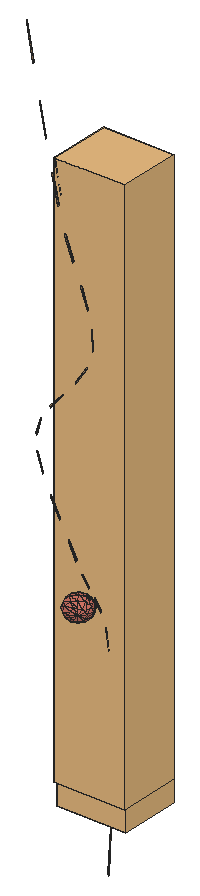
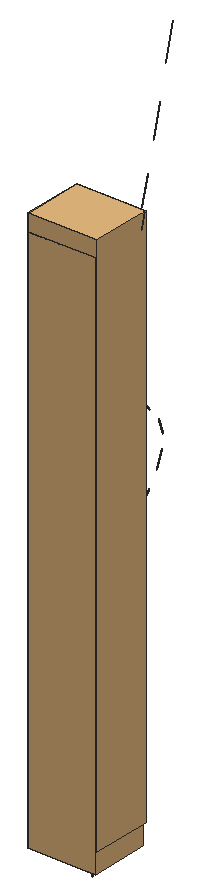
# SketchUp Ruby script. Lengths in inches.
U = 1.inch
M = Sketchup.active_model
def pt(a) = Geom::Point3d.new(a.map { |v| v * U })
def face(e, loops, mat)
  f = e.add_face(loops[0].map { |a| pt(a) })
  loops[1..].each { |l| e.add_face(l.map { |a| pt(a) }).erase! }
  f.material = f.back_material = mat if mat
  f
end
# faces: each face lists its corners as indices into pts; further lists are holes
def faces(e, pts, list, mat = nil) = list.each { |f| face(e, (f[0].is_a?(Array) ? f : [f]).map { |l| l.map { |i| pts[i] } }, mat) }
# xy, xz, yz: faces in a plane at the given z, y or x. An outline is a flat list of corners, or four numbers for a rectangle; further outlines are holes
def ring(l) = l.size == 4 ? [[l[0], l[1]], [l[2], l[1]], [l[2], l[3]], [l[0], l[3]]] : l.each_slice(2).to_a
def flat(e, list, mat, &to3) = list.each { |f| face(e, (f[0].is_a?(Array) ? f : [f]).map { |l| ring(l).map { |u, v| to3.(u, v) } }, mat) }
def xy(e, z, list, mat = nil) = flat(e, list, mat) { |x, y| [x, y, z] }
def xz(e, y, list, mat = nil) = flat(e, list, mat) { |x, z| [x, y, z] }
def yz(e, x, list, mat = nil) = flat(e, list, mat) { |y, z| [x, y, z] }
def lines(e, pts, list) = list.each { |a, b| e.add_line(pt(pts[a]), pt(pts[b])) }
# prism: a flat outline (further loops are holes) pulled along v
def prism(e, loops, v, mat = nil)
  f = face(e, loops, mat); d = Geom::Vector3d.new(v.map { |x| x * U })
  f.pushpull(f.normal.samedirection?(d) ? d.length : -d.length)
end
def box(e, o, s, mat = nil) = prism(e, [[o, [o[0] + s[0], o[1], o[2]], [o[0] + s[0], o[1] + s[1], o[2]], [o[0], o[1] + s[1], o[2]]]], [0, 0, s[2]], mat)
def at(x, y, z, deg = 0) = Geom::Transformation.translation(pt([x, y, z])) * Geom::Transformation.rotation(ORIGIN, Z_AXIS, deg.degrees)
def axes(o, x, y, z) = Geom::Transformation.new([*x, 0, *y, 0, *z, 0, *pt(o).to_a, 1])
def part(name) = M.definitions.add(name)
# library, detail: a bought-in or finely detailed component or shape, given as its bounding box
def library(name, o, s) = part(name).tap { |d| box(d.entities, o, s) }
def detail(e, o, s) = box(e.add_group.entities, o, s)
def put(e, d, t, mat = nil) = e.add_instance(d, t).tap { |i| i.material = mat if mat }
def group(e, t, mat = nil) = e.add_group.tap { |g| g.transformation = t; g.material = mat if mat }.entities
root = M.entities
M.materials.add("green").color = [174, 139, 102]
M.materials.add("vio").color = [206, 114, 100]
c1 = part("3DGeom~157_Defintion")
p = [[36.26,422.52,-32.42],[38.24,377.08,-31.875],[36.84,377.08,-32.625],[36.48,335.72,-32.39],[36.5,298.41,-30.99],[35.18,298.44,-31.7],
  [37.84,335.71,-31.66],[37.69,422.54,-31.65],[32.26,525.68,-30.66],[36.2,472.09,-30.97],[34.73,472.06,-31.76],[33.77,525.72,-29.85],
  [38.91,422.55,-30.49],[40.28,377.08,-29.35],[39.43,377.08,-30.75],[32.92,265.24,-30.5625],[30.44,237.94,-28.41],[29.19,238.08,-29.09],
  [34.2,265.18,-29.87],[39,335.7,-30.56],[38.43,298.38,-28.59],[37.62,298.39,-29.92],[39,335.7,-30.56],[39.83,335.69,-29.19],
  [38.91,422.55,-30.49],[39.79,422.55,-29.05],[35.05,525.75,-28.63],[38.35,472.11,-28.31],[37.45,472.11,-29.79],[35.3,265.14,-28.83],
  [32.28,237.79,-26.11],[31.51,237.83,-27.38],[35.3,265.14,-28.83],[36.08,265.13,-27.54],[35.05,525.75,-28.63],[35.97,525.76,-27.12],
  [23.82,217.46,-27.21],[18.65,200.68,-24.19],[17.48,200.96,-24.87],[25.03,217.22,-26.53],[26.07,217.0625,-25.51],[20.4,200.41,-21.9375],
  [19.66,200.49,-23.18],[26.07,217.0625,-25.51],[26.82,216.99,-24.25],[10.9,186.23,-22.05],[5.93,170.61,-18.08],[4.76,170.8,-18.73],
  [12.06,185.96,-21.38],[13.07,185.79,-20.39],[7.7,170.5,-15.93],[6.95,170.51,-17.12],[13.07,185.79,-20.39],[13.8,185.74,-19.17],
  [20.05,-83.49,-19.57],[20.36,-107.02,-19.07],[19.4,-106.97,-19.5],[21.05,-83.47,-19.125],[21.92,-83.48,-18.41],[21.84,-107.05,-17.47],
  [21.21,-107.04,-18.37],[21.92,-83.48,-18.41],[22.57,-83.5,-17.49],[15.89,-132.25,-16.89],[11.4,-159.71,-12.15],[10.49,-159.62,-12.57],
  [16.82,-132.33,-16.46],[17.65,-132.37,-15.78],[12.79,-159.74,-10.65],[12.19,-159.75,-11.49],[17.65,-132.37,-15.78],[18.26,-132.36,-14.91],
  [8.68,-47.13,-7.48],[17.3,-62.98,-14.9375],[16.31,-63.1,-15.41],[9.65,-46.9375,-6.96],[-0.37,152.09,-14.84],[-4.1,128.9,-8.55],
  [-5.27,128.96,-9.15],[0.82,152,-14.22],[10.53,-46.89,-6.21],[18.84,-63.04,-13.28],[18.18,-62.96,-14.21],[10.53,-46.89,-6.21],
  [11.23,-47.01,-5.28],[1.84,151.98,-13.29],[-2.34,129.04,-6.52],[-3.09,128.93,-7.65],[1.84,151.98,-13.29],[2.59,152.03,-12.12],
  [4.13,-189.34,-7.37],[-1.4,-221.72,-1.7],[-2.26,-221.65,-2.09],[5.01,-189.42,-6.97],[5.79,-189.46,-6.32],[-0.09,-221.74,-0.28],
  [-0.65,-221.75,-1.08],[5.79,-189.46,-6.32],[6.37,-189.45,-5.5],[-10.47,103.92,-1.64],[-14.15,78.09,6.94],[-15.28,78.11,6.38],
  [-9.3125,103.88,-1.06],[-8.3125,103.93,-0.18],[-12.43,78.3,8.88],[-13.16,78.16,7.8],[-8.3125,103.93,-0.18],[-7.57,104.07,0.93],
  [-9.84,-21.39,10.9375],[0.27,-33.63,2.53],[-0.69,-33.86,1.98],[-7.77,-256.8,2.46],[-11.81,-294.96,6.87],[-12.6,-294.92,6.51],
  [-6.94,-256.85,2.84],[-8.85,-21.17,11.49],[-7.96,-21.11,12.28],[1.87,-33.69,4.24],[1.16,-33.57,3.31],[-6.21,-256.87,3.44],
  [-10.59,-294.97,8.17],[-11.11,-294.98,7.4375],[-6.21,-256.87,3.44],[-5.66,-256.86,4.21],[-7.96,-21.11,12.28],[-7.25,-21.21,13.24],
  [-17.49,-335.72,10.65],[-21.71,-379.24,15.19],[-22.42,-379.2,14.875],[-16.73,-335.76,10.98],[-16.07,-335.78,11.53],[-20.62,-379.24,16.37],
  [-21.08,-379.25,15.71],[-16.07,-335.78,11.53],[-15.58,-335.77,12.22],[-19.05,52.72,13.59],[-20.01,29.02,19.21],[-21.11,28.99,18.68],
  [-17.94,52.72,14.13],[-16.97,52.79,14.98],[-18.37,29.18,21.08],[-19.0625,29.08,20.03],[-16.97,52.79,14.98],[-16.26,52.93,16.03],
  [-20.8125,8.25,20.38],[-15.98,-7.82,18.1],[-17.02,-7.99,17.57],[-19.74,8.3125,20.9],[-18.81,8.36,21.71],[-14.38,-7.82,19.9],
  [-15.07,-7.76,18.9],[-27.41,-425.36,19.19],[-31.82,-474.23,23.89],[-32.45,-474.2,23.61],[-26.74,-425.39,19.5],[-18.81,8.36,21.71],
  [-18.13,8.38,22.74],[-26.15,-425.41,19.98],[-30.85,-474.24,24.93],[-31.27,-474.24,24.35],[-26.15,-425.41,19.98],[-25.71,-425.4,20.6]]
faces(c1.entities,p,[[0,1,2],[3,4,5],[3,6,4],[0,7,1],[8,9,10],[8,11,9],[12,13,14],[15,16,17],
  [15,18,16],[19,20,21],[22,23,20],[24,25,13],[26,27,28],[29,30,31],[32,33,30],[34,35,27],
  [36,37,38],[36,39,37],[40,41,42],[43,44,41],[45,46,47],[45,48,46],[49,50,51],[52,53,50],
  [54,55,56],[54,57,55],[58,59,60],[61,62,59],[63,64,65],[63,66,64],[67,68,69],[70,71,68],
  [72,73,74],[72,75,73],[76,77,78],[76,79,77],[80,81,82],[83,84,81],[85,86,87],[88,89,86],
  [90,91,92],[90,93,91],[94,95,96],[97,98,95],[99,100,101],[99,102,100],[103,104,105],[106,107,104],
  [108,109,110],[111,112,113],[111,114,112],[108,115,109],[116,117,118],[119,120,121],[122,123,120],[124,125,117],
  [126,127,128],[126,129,127],[130,131,132],[133,134,131],[135,136,137],[135,138,136],[139,140,141],[142,143,140],
  [144,145,146],[144,147,145],[148,149,150],[151,152,153],[151,154,152],[155,156,149],[157,158,159],[160,161,158]],"green")
c2 = part("3DGeom~246_Defintion")
p = [[52.16,0,-500],[255.625,-213.37,-352.41],[17.91,-184.79,-452.79],[295.17,0,-406.93],[-204.83,0,-459.09],[-224.6,106.69,-431.83],
  [17.91,184.79,-452.79],[-224.6,-106.6875,-431.83],[-406.93,0,-295.17],[-406.93,0,-295.17],[147.59,-369.57,-203.47],[-75.65,-320.06,-323.79],
  [147.59,-369.57,-203.47],[-75.65,-320.06,-323.79],[255.625,213.37,-352.41],[-278.62,184.79,-357.36],[-75.65,320.06,-323.79],[-75.65,-320.06,-323.79],
  [-278.62,-184.79,-357.36],[-278.62,-184.79,-357.36],[-406.93,0,-295.17],[-406.93,0,-295.17],[295.17,0,-406.93],[424.85,-184.79,-157.61],
  [255.625,-213.37,-352.41],[295.17,0,-406.93],[459.09,0,-204.83],[255.625,213.37,-352.41],[295.17,0,-406.93],[-278.62,-184.79,-357.36],
  [-203.47,-369.57,-147.59],[-352.41,-213.37,-255.625],[-278.62,-184.79,-357.36],[-75.65,-320.06,-323.79],[-278.62,-184.79,-357.36],[-352.41,-213.37,-255.625],
  [-406.93,0,-295.17],[-352.41,213.37,-255.625],[-278.62,184.79,-357.36],[-352.41,213.37,-255.625],[-75.65,320.06,-323.79],[-278.62,184.79,-357.36],
  [255.625,-213.37,-352.41],[331.28,-320.06,-28.62],[147.59,-369.57,-203.47],[255.625,-213.37,-352.41],[331.28,-320.06,-28.62],[255.625,213.37,-352.41],
  [424.85,184.79,-157.61],[147.59,369.57,-203.47],[255.625,213.37,-352.41],[147.59,369.57,-203.47],[0,-426.74,0],[147.59,-369.57,-203.47],
  [-352.41,213.37,-255.625],[-203.47,369.57,-147.59],[-75.65,320.06,-323.79],[147.59,369.57,-203.47],[-75.65,320.06,-323.79],[-426.21,-184.79,-153.89],
  [-480.23,-106.6875,-79.42],[-500,0,-52.16],[-480.23,106.6875,-79.42],[-426.21,184.78,-153.89],[-203.47,-369.57,-147.59],[-331.28,-320.06,28.62],
  [-203.47,369.57,-147.59],[480.23,-106.69,79.42],[500,0,52.16],[203.47,-369.57,147.59],[331.28,-320.06,-28.62],[147.59,369.57,-203.47],
  [331.28,320.06,-28.62],[0,426.74,0],[331.28,320.06,-28.62],[147.59,369.57,-203.47],[147.59,369.57,-203.47],[426.21,-184.78,153.89],
  [331.28,-320.06,-28.62],[480.23,106.6875,79.42],[-424.85,-184.78,157.61],[-331.28,320.06,28.62],[-203.47,369.57,-147.59],[-147.59,-369.57,203.47],
  [-147.59,-369.57,203.47],[-331.28,-320.06,28.62],[-331.28,320.06,28.62],[-459.09,0,204.83],[-424.85,184.79,157.61],[331.28,-320.06,-28.62],
  [352.41,-213.37,255.625],[203.47,-369.57,147.59],[331.28,-320.06,-28.62],[426.21,184.79,153.89],[203.47,369.57,147.59],[203.47,369.57,147.59],
  [331.28,320.06,-28.62],[75.65,-320.06,323.79],[-147.59,-369.57,203.47],[75.65,-320.06,323.79],[-331.28,320.06,28.62],[-147.59,369.57,203.47],
  [-147.59,-369.57,203.47],[-255.625,-213.37,352.41],[-147.59,369.57,203.47],[406.93,0,295.17],[278.62,-184.79,357.36],[75.65,-320.06,323.79],
  [352.41,-213.37,255.625],[278.62,-184.79,357.36],[203.47,369.57,147.59],[352.41,213.37,255.625],[75.65,320.06,323.79],[352.41,213.37,255.625],
  [-295.17,0,406.93],[-255.625,213.37,352.41],[-147.59,369.57,203.47],[-147.59,-369.57,203.47],[-17.91,-184.79,452.79],[-255.625,-213.37,352.41],
  [-147.59,-369.57,203.47],[75.65,-320.06,323.79],[-255.625,213.37,352.41],[75.65,320.06,323.79],[-147.59,369.57,203.47],[278.62,-184.79,357.36],
  [278.62,184.79,357.36],[278.62,184.79,357.36],[352.41,213.37,255.625],[224.6,-106.69,431.83],[278.62,-184.79,357.36],[406.93,0,295.17],
  [204.83,0,459.09],[406.93,0,295.17],[224.6,106.6875,431.83],[406.93,0,295.17],[278.62,184.79,357.36],[406.93,0,295.17],
  [-255.625,213.37,352.41],[-17.91,184.79,452.79],[75.65,320.06,323.79],[278.62,184.79,357.36],[75.65,320.06,323.79],[-255.625,-213.37,352.41],
  [-52.16,0,500],[-295.17,0,406.93],[-255.625,-213.37,352.41],[-295.17,0,406.93],[-255.625,213.37,352.41],[278.62,184.79,357.36],
  [-295.17,0,406.93]]
faces(c2.entities,p,[[0,1,2],[0,3,1],[4,0,2],[5,6,0],[5,0,4],[6,3,0],[4,2,7],[4,7,8],
  [5,4,9],[2,10,11],[2,1,12],[7,2,13],[6,14,3],[15,6,5],[15,16,6],[16,14,6],
  [7,17,18],[7,19,20],[15,5,21],[22,23,24],[25,26,23],[27,26,28],[29,30,31],[32,33,30],
  [34,35,36],[37,38,36],[39,40,41],[42,43,44],[45,23,46],[47,48,26],[49,48,50],[16,51,14],
  [33,52,30],[33,53,52],[54,55,56],[55,57,58],[35,59,36],[59,60,36],[60,61,36],[61,62,36],
  [62,63,36],[63,37,36],[35,64,65],[35,65,59],[63,66,37],[26,67,23],[26,68,67],[48,68,26],
  [53,69,52],[53,70,69],[71,72,48],[73,74,75],[55,73,76],[23,77,78],[23,67,77],[48,79,68],
  [72,79,48],[59,65,80],[59,80,60],[62,81,63],[63,81,82],[30,52,83],[30,84,85],[86,73,55],
  [60,80,87],[60,87,61],[61,88,62],[62,88,81],[61,87,88],[89,90,91],[92,77,90],[72,93,79],
  [94,93,72],[73,95,96],[52,97,98],[52,69,99],[100,101,73],[101,95,73],[65,102,103],[65,103,80],
  [88,104,81],[67,68,105],[68,79,105],[77,67,105],[79,93,105],[69,106,107],[69,108,109],[110,111,93],
  [112,113,95],[101,112,95],[90,77,105],[93,111,105],[80,103,114],[80,114,87],[87,115,88],[88,115,116],
  [117,118,119],[120,121,118],[122,123,124],[87,114,115],[125,90,105],[111,126,105],[112,127,128],[129,130,131],
  [132,129,133],[134,132,135],[136,134,137],[121,129,118],[121,130,129],[138,139,140],[139,141,142],[143,144,145],
  [146,118,144],[147,139,148],[139,134,149],[150,144,139],[118,129,132],[144,132,134],[144,134,139],[118,132,144]],"vio")
c3 = part("3DGeom~39_Defintion")
p = [[35.12,-55.5,-54.41],[34.11,-55.53,-54.86],[35.81,-76.47,-55.34],[36.8,-76.41,-54.9],[38.88,-99.33,-54.67],[37.91,-99.4,-55.11],
  [39.32,-123.69,-53.625],[40.28,-123.64,-53.2],[37.08,-24.79,-53.05],[36.07,-24.5,-53.5],[33.89,-37.16,-54.23],[34.93,-37.21,-53.77],
  [44.64,-14.39,-49.98],[39.94,-17.85,-52.2],[40.77,-18.46,-51.8125],[43.83,-13.75,-50.35],[39.93,-148.71,-49.9375],[38.99,-148.72,-50.36],
  [35.86,-173.84,-44.78],[36.78,-173.89,-44.36],[49.18,2.9,-43.4],[46.875,-8.22,-47.77],[47.86,-8.59,-47.26],[48.17,3.01,-43.99],
  [40.94,55.6,-31.2],[39.91,55.54,-31.86],[46.25,23.72,-38.95],[47.26,23.73,-38.32],[29.9,-199.58,-35.34],[29.03,-199.5,-35.76],
  [19.05,-226.47,-23.39],[19.9,-226.57,-22.96],[18.98,142.12,-11.91],[17.89,142.02,-12.62],[29.92,96.01,-22.77],[30.98,96.1,-22.08],
  [8.08,-254.51,-8.72],[7.27,-254.41,-9.13],[-4.99,-283,5.49],[-4.2,-283.09,5.89],[-4.75,238.47,7.76],[-5.91,238.39,7],
  [5.41,190.5,-2.38],[6.54,190.59,-1.65],[-19.28,323.69,21.26],[-20.52,323.65,20.47],[-14.48,282.67,14.58],[-13.28,282.72,15.35],
  [-15.6,-312.05,19.375],[-16.37,-311.96,18.99],[-25.53,-341.05,29.86],[-24.78,-341.11,30.22],[-27.78,403.71,30.46],[-29.08,403.69,29.63],
  [-25.39,363.99,25.48],[-24.12,364.02,26.29],[-31.6,481.16,36.19],[-32.96,481.18,35.32],[-31.61,442.75,32.91],[-30.28,442.76,33.76],
  [-31.87,-370.06,38.59],[-32.6,-370.01,38.24],[-38.75,-399.23,45.4375],[-38.04,-399.28,45.77],[-43.3,-428.76,51.78],[-43.98,-428.72,51.46],
  [-48.3,-458.49,56.3],[-47.64,-458.51,56.62],[-51.06,-488.54,60.27],[-51.7,-488.51,59.97],[-54.18,-518.81,62.46],[-53.57,-518.82,62.75]]
faces(c3.entities,p,[[0,1,2],[0,2,3],[4,5,6],[4,6,7],[8,9,10],[8,10,11],[12,13,14],[12,15,13],
  [16,17,18],[16,18,19],[20,21,22],[20,23,21],[24,25,26],[24,26,27],[28,29,30],[28,30,31],
  [32,33,34],[32,34,35],[36,37,38],[36,38,39],[40,41,42],[40,42,43],[44,45,46],[44,46,47],
  [48,49,50],[48,50,51],[52,53,54],[52,54,55],[56,57,58],[56,58,59],[60,61,62],[60,62,63],
  [64,65,66],[64,66,67],[68,69,70],[68,70,71]],"green")
c4 = part("3DGeom~43_Defintion")
p = [[34.1,-55.53,-54.86],[33.24,-55.55,-55.5625],[34.97,-76.52,-56.03],[34.97,-76.52,-56.03],[35.81,-76.47,-55.34],[37.9,-99.39,-55.1],
  [37.08,-99.46,-55.78],[38.51,-123.75,-54.29],[38.51,-123.75,-54.29],[39.32,-123.6875,-53.625],[36.18,-55.46,-54.25],[35.12,-55.5,-54.41],
  [36.8,-76.4,-54.89],[37.84,-76.34,-54.74],[36.07,-24.5,-53.5],[33.01,-37.11,-54.9375],[33.89,-37.16,-54.22],[35.22,-24.22,-54.2],
  [33.01,-37.11,-54.9375],[39.9,-99.26,-54.51],[38.875,-99.33,-54.67],[40.28,-123.64,-53.2],[41.28,-123.61,-53.04],[38.13,-25.08,-52.89],
  [34.92,-37.21,-53.77],[36.01,-37.26,-53.6],[37.08,-24.79,-53.05],[43.83,-13.75,-50.35],[39.26,-17.27,-52.85],[39.94,-17.85,-52.2],
  [43.19,-13.12,-50.98],[39.26,-17.27,-52.85],[45.52,-14.98,-49.89],[40.76,-18.46,-51.81],[41.65,-19.04,-51.71],[44.63,-14.39,-49.98],
  [38.99,-148.71,-50.36],[38.2,-148.76,-51.01],[35.09,-173.85,-45.42],[35.09,-173.85,-45.42],[35.86,-173.83,-44.78],[40.91,-148.73,-49.78],
  [39.93,-148.7,-49.9375],[36.77,-173.88,-44.35],[37.72,-173.98,-44.18],[48.17,3.01,-43.99],[46.09,-7.82,-48.51],[46.875,-8.22,-47.76],
  [48.17,3.01,-43.99],[47.35,3.18,-44.83],[50.28,2.84,-43.09],[47.85,-8.59,-47.25],[48.92,-8.89,-47.03],[49.18,2.9,-43.39],
  [39.91,55.53,-31.86],[45.4375,23.76,-39.82],[46.25,23.72,-38.95],[39.91,55.53,-31.86],[39.08,55.54,-32.77],[42.07,55.72,-30.83],
  [40.94,55.6,-31.2],[47.26,23.73,-38.3125],[48.36,23.79,-37.97],[29.03,-199.49,-35.76],[28.28,-199.5,-36.39],[18.33,-226.47,-24],
  [18.33,-226.47,-24],[19.05,-226.46,-23.38],[30.81,-199.72,-35.15],[29.9,-199.57,-35.34],[19.9,-226.56,-22.96],[20.77,-226.74,-22.76],
  [17.89,142.02,-12.62],[17.01,142,-13.59],[29.07,96,-23.71],[17.89,142.02,-12.62],[29.92,96.01,-22.77],[20.17,142.27,-11.51],
  [18.98,142.11,-11.91],[30.98,96.09,-22.07],[32.14,96.24,-21.69],[7.27,-254.4,-9.13],[6.56,-254.4,-9.73],[-5.67,-282.99,4.91],
  [-5.67,-282.99,4.91],[-4.99,-282.98,5.49],[8.92,-254.68,-8.52],[8.08,-254.5,-8.72],[-4.2,-283.08,5.89],[-3.38,-283.26,6.08],
  [-5.91,238.375,7],[-6.85,238.36,5.97],[4.51,190.47,-3.39],[-5.91,238.375,7],[5.41,190.49,-2.38],[-3.48,238.6,8.17],
  [-4.75,238.46,7.76],[6.54,190.58,-1.65],[7.77,190.74,-1.24],[-20.52,323.63,20.47],[-21.51,323.64,19.38],[-15.45,282.66,13.52],
  [-20.52,323.63,20.47],[-14.48,282.65,14.58],[-17.93,323.76,21.68],[-19.28,323.68,21.26],[-13.28,282.71,15.35],[-11.96,282.8125,15.77],
  [-16.37,-311.95,18.99],[-17.03,-311.95,18.43],[-26.16,-341.03,29.3125],[-26.16,-341.03,29.3125],[-25.53,-341.03,29.86],[-14.8,-312.18,19.55],
  [-15.6,-312.03,19.375],[-24.78,-341.09,30.22],[-23.99,-341.2,30.375],[-29.08,403.67,29.63],[-30.12,403.6875,28.5],[-26.4,363.98,24.37],
  [-29.08,403.67,29.63],[-25.39,363.97,25.48],[-26.36,403.74,30.9],[-27.78,403.6875,30.46],[-24.12,364,26.29],[-22.73,364.07,26.72],
  [-32.96,481.15,35.32],[-32.67,442.75,31.75],[-31.61,442.73,32.91],[-32.96,481.15,35.32],[-34.05,481.18,34.13],[-30.11,481.14,36.64],
  [-31.6,481.14,36.18],[-30.28,442.73,33.76],[-28.82,442.76,34.2],[-32.6,-369.99,38.23],[-33.21,-369.99,37.71],[-39.34,-399.21,44.93],
  [-39.34,-399.21,44.93],[-38.75,-399.21,45.43],[-31.11,-370.14,38.73],[-31.87,-370.04,38.58],[-38.04,-399.25,45.77],[-37.3,-399.34,45.91],
  [-43.98,-428.7,51.46],[-44.55,-428.7,50.97],[-48.85,-458.46,55.83],[-48.85,-458.46,55.83],[-48.3,-458.46,56.3],[-42.58,-428.8,51.91],
  [-43.3,-428.74,51.78],[-47.64,-458.49,56.61],[-46.95,-458.54,56.74],[-51.7,-488.49,59.97],[-52.23,-488.48,59.51],[-54.6875,-518.78,62.02],
  [-54.6875,-518.78,62.02],[-54.18,-518.78,62.46],[-50.4,-488.55,60.39],[-51.0625,-488.51,60.27],[-53.57,-518.8,62.75],[-52.93,-518.82,62.86]]
faces(c4.entities,p,[[0,1,2],[0,3,4],[5,6,7],[5,8,9],[10,11,12],[10,12,13],[14,15,16],[14,17,18],
  [19,20,21],[19,21,22],[23,24,25],[23,26,24],[27,28,29],[27,30,31],[32,33,34],[32,35,33],
  [36,37,38],[36,39,40],[41,42,43],[41,43,44],[45,46,47],[48,49,46],[50,51,52],[50,53,51],
  [54,55,56],[57,58,55],[59,60,61],[59,61,62],[63,64,65],[63,66,67],[68,69,70],[68,70,71],
  [72,73,74],[75,74,76],[77,78,79],[77,79,80],[81,82,83],[81,84,85],[86,87,88],[86,88,89],
  [90,91,92],[93,92,94],[95,96,97],[95,97,98],[99,100,101],[102,101,103],[104,105,106],[104,106,107],
  [108,109,110],[108,111,112],[113,114,115],[113,115,116],[117,118,119],[120,119,121],[122,123,124],[122,124,125],
  [126,127,128],[129,130,127],[131,132,133],[131,133,134],[135,136,137],[135,138,139],[140,141,142],[140,142,143],
  [144,145,146],[144,147,148],[149,150,151],[149,151,152],[153,154,155],[153,156,157],[158,159,160],[158,160,161]],"green")
c5 = part("3DGeom~38_Defintion")
p = [[36.53,-75.84,-54.49],[35.54,-75.9,-54.93],[37.625,-98.66,-54.7],[38.59,-98.59,-54.27],[34.67,-36.9375,-53.37],[33.64,-36.89,-53.82],
  [33.85,-55.12,-54.46],[34.86,-55.09,-54.01],[39.98,-122.72,-52.8],[39.03,-122.77,-53.23],[38.7,-147.61,-49.99],[40.46,-18.32,-51.43],
  [35.81,-24.32,-53.1],[36.81,-24.61,-52.65],[39.64,-17.72,-51.8125],[39.63,-147.6,-49.57],[47.5,-8.52,-46.91],[43.5,-13.65,-49.98],
  [44.3,-14.29,-49.61],[46.53,-8.16,-47.41],[36.5,-172.59,-44.03],[35.6,-172.55,-44.45],[28.8125,-198.01,-35.5],[29.68,-198.09,-35.07],
  [46.91,23.55,-38.03],[47.81,2.99,-43.67],[48.82,2.875,-43.07],[45.91,23.54,-38.66],[30.75,95.38,-21.91],[29.7,95.3,-22.6],
  [39.61,55.12,-31.625],[40.64,55.18,-30.97],[19.75,-224.88,-22.79],[18.91,-224.79,-23.21],[7.21,-252.52,-9.07],[8.02,-252.62,-8.65],
  [6.49,189.18,-1.63],[5.37,189.08,-2.36],[17.76,140.97,-12.53],[18.84,141.0625,-11.82],[-4.17,-280.99,5.85],[-4.95,-280.89,5.45],
  [-16.25,-309.64,18.85],[-15.49,-309.73,19.23],[-13.18,280.62,15.24],[-14.375,280.56,14.47],[-5.87,236.61,6.95],[-4.71,236.7,7.7],
  [-23.9375,361.3125,26.1],[-25.2,361.28,25.3],[-20.37,321.24,20.31],[-19.14,321.29,21.1],[-30.05,439.46,33.51],[-31.375,439.46,32.67],
  [-28.87,400.6875,29.41],[-27.58,400.7,30.23],[-24.59,-338.57,30],[-25.34,-338.51,29.63],[-32.35,-367.25,37.95],[-31.63,-367.31,38.3],
  [-31.52,515.07,37.46],[-32.9,515.1,36.59],[-32.72,477.6,35.0625],[-31.37,477.58,35.92],[-37.76,-396.3,45.43],[-38.46,-396.26,45.1],
  [-43.65,-425.53,51.08],[-42.98,-425.57,51.4],[-47.29,-455.1,56.19],[-47.9375,-455.07,55.89],[-51.3125,-484.88,59.53],[-50.68,-484.9,59.82]]
faces(c5.entities,p,[[0,1,2],[0,2,3],[4,5,6],[4,6,7],[8,9,10],[11,12,13],[11,14,12],[8,10,15],
  [16,17,18],[16,19,17],[20,21,22],[20,22,23],[24,25,26],[24,27,25],[28,29,30],[28,30,31],
  [32,33,34],[32,34,35],[36,37,38],[36,38,39],[40,41,42],[40,42,43],[44,45,46],[44,46,47],
  [48,49,50],[48,50,51],[52,53,54],[52,54,55],[56,57,58],[56,58,59],[60,61,62],[60,62,63],
  [64,65,66],[64,66,67],[68,69,70],[68,70,71]],"green")
c6 = part("3DGeom~41_Defintion")
p = [[35.54,-75.9,-54.92],[34.7,-75.95,-55.61],[36.8,-98.72,-55.36],[36.8,-98.72,-55.36],[37.62,-98.65,-54.69],[33.64,-36.88,-53.82],
  [32.76,-36.83,-54.53],[33,-55.14,-55.15],[33,-55.14,-55.15],[33.85,-55.12,-54.45],[37.55,-75.77,-54.33],[36.52,-75.83,-54.49],
  [38.59,-98.59,-54.26],[39.6,-98.52,-54.11],[35.74,-36.98,-53.2],[34.66,-36.93,-53.37],[34.86,-55.09,-54.01],[35.91,-55.05,-53.84],
  [39.03,-122.76,-53.22],[38.22,-122.82,-53.88],[37.91,-147.65,-50.63],[39.64,-17.72,-51.81],[34.96,-24.04,-53.8],[35.8,-24.32,-53.1],
  [38.97,-17.14,-52.46],[34.96,-24.04,-53.8],[37.91,-147.65,-50.63],[38.7,-147.6,-49.98],[40.97,-122.6875,-52.65],[39.97,-122.72,-52.8],
  [39.63,-147.59,-49.5625],[41.34,-18.9,-51.33],[36.8,-24.61,-52.65],[37.85,-24.89,-52.5],[40.46,-18.32,-51.42],[40.6,-147.62,-49.41],
  [46.52,-8.16,-47.41],[42.87,-13.02,-50.6],[43.5,-13.65,-49.97],[45.74,-7.77,-48.15],[42.87,-13.02,-50.6],[48.56,-8.83,-46.68],
  [44.3,-14.29,-49.6],[45.18,-14.87,-49.52],[47.5,-8.52,-46.9],[35.6,-172.54,-44.45],[34.83,-172.56,-45.08],[28.07,-198.01,-36.12],
  [45.91,23.54,-38.65],[47,3.16,-44.49],[47.81,2.99,-43.66],[45.91,23.54,-38.65],[45.1,23.59,-39.52],[28.07,-198.01,-36.12],
  [28.8125,-198,-35.5],[37.44,-172.68,-43.85],[36.5,-172.58,-44.02],[29.68,-198.08,-35.07],[30.58,-198.23,-34.88],[48,23.61,-37.69],
  [48.8125,2.875,-43.07],[49.91,2.82,-42.76],[46.91,23.55,-38.03],[29.7,95.29,-22.6],[28.85,95.28,-23.53],[38.79,55.13,-32.53],
  [29.7,95.29,-22.6],[39.61,55.12,-31.625],[31.9,95.53,-21.53],[30.75,95.375,-21.91],[40.64,55.18,-30.96],[41.75,55.31,-30.6],
  [18.91,-224.77,-23.21],[18.19,-224.78,-23.82],[6.52,-252.5,-9.66],[6.52,-252.5,-9.66],[7.21,-252.5,-9.07],[20.61,-225.05,-22.59],
  [19.75,-224.87,-22.79],[8.02,-252.6,-8.65],[8.86,-252.78,-8.46],[5.37,189.07,-2.36],[4.47,189.05,-3.36],[16.88,140.94,-13.49],
  [5.37,189.07,-2.36],[17.75,140.96,-12.53],[7.71,189.32,-1.23],[6.49,189.16,-1.63],[18.84,141.05,-11.82],[20.02,141.21,-11.43],
  [-4.95,-280.875,5.45],[-5.63,-280.875,4.875],[-16.9,-309.625,18.29],[-16.9,-309.625,18.29],[-16.25,-309.62,18.85],[-3.36,-281.15,6.04],
  [-4.17,-280.97,5.85],[-15.49,-309.7,19.23],[-14.375,280.54,14.47],[-15.33,280.55,13.42],[-6.79,236.59,5.92],[-14.375,280.54,14.47],
  [-5.87,236.6,6.95],[-14.69,-309.86,19.4],[-11.87,280.7,15.65],[-13.18,280.6,15.24],[-4.71,236.68,7.7],[-3.45,236.82,8.11],
  [-25.2,361.26,25.29],[-26.2,361.27,24.19],[-21.35,321.23,19.24],[-25.2,361.26,25.29],[-20.37,321.22,20.3125],[-22.5625,361.36,26.52],
  [-23.9375,361.29,26.09],[-19.14,321.26,21.1],[-17.8,321.35,21.52],[-31.37,439.43,32.67],[-32.43,439.45,31.51],[-29.9,400.68,28.28],
  [-31.37,439.43,32.67],[-28.87,400.66,29.41],[-25.34,-338.49,29.63],[-25.97,-338.49,29.09],[-32.96,-367.23,37.43],[-32.96,-367.23,37.43],
  [-32.35,-367.23,37.95],[-23.81,-338.66,30.15],[-24.59,-338.55,29.99],[-31.63,-367.28,38.3],[-30.875,-367.375,38.44],[-28.61,439.46,33.95],
  [-30.05,439.43,33.5],[-27.58,400.68,30.23],[-26.16,400.72,30.67],[-32.9,515.0625,36.59],[-34,515.1,35.38],[-33.79,477.59,33.88],
  [-32.9,515.0625,36.59],[-32.72,477.5625,35.06],[-30,515.01,37.92],[-31.51,515.03,37.46],[-31.36,477.55,35.91],[-29.89,477.55,36.37],
  [-38.46,-396.23,45.09],[-39.05,-396.23,44.59],[-44.22,-425.5,50.59],[-44.22,-425.5,50.59],[-43.65,-425.5,51.07],[-37.03,-396.36,45.57],
  [-37.76,-396.28,45.43],[-42.98,-425.54,51.39],[-42.27,-425.61,51.52],[-47.9375,-455.04,55.88],[-48.48,-455.04,55.41],[-51.84,-484.84,59.07],
  [-51.84,-484.84,59.07],[-51.31,-484.84,59.52],[-46.6,-455.12,56.3125],[-47.28,-455.07,56.19],[-50.68,-484.87,59.82],[-50.02,-484.9,59.9375]]
faces(c6.entities,p,[[0,1,2],[0,3,4],[5,6,7],[5,8,9],[10,11,12],[10,12,13],[14,15,16],[14,16,17],
  [18,19,20],[21,22,23],[21,24,25],[18,26,27],[28,29,30],[31,32,33],[31,34,32],[28,30,35],
  [36,37,38],[36,39,40],[41,42,43],[41,44,42],[45,46,47],[48,49,50],[51,52,49],[45,53,54],
  [55,56,57],[55,57,58],[59,60,61],[59,62,60],[63,64,65],[66,65,67],[68,69,70],[68,70,71],
  [72,73,74],[72,75,76],[77,78,79],[77,79,80],[81,82,83],[84,83,85],[86,87,88],[86,88,89],
  [90,91,92],[90,93,94],[95,96,97],[98,99,100],[101,100,102],[95,97,103],[104,105,106],[104,106,107],
  [108,109,110],[111,110,112],[113,114,115],[113,115,116],[117,118,119],[120,119,121],[122,123,124],[122,125,126],
  [127,128,129],[127,129,130],[131,132,133],[131,133,134],[135,136,137],[138,137,139],[140,141,142],[140,142,143],
  [144,145,146],[144,147,148],[149,150,151],[149,151,152],[153,154,155],[153,156,157],[158,159,160],[158,160,161]],"green")
c7 = library("3DGeom~45_Defintion",[-55.29,-518.75,-62.82],[110.58,1000,125.64])
c8 = library("3DGeom~42_Defintion",[-55.29,-518.75,-62.82],[110.58,1000,125.58])
c9 = library("3DGeom~44_Defintion",[-52.47,-485.07,-62.35],[107.35,1000,122.25])
c10 = library("3DGeom~40_Defintion",[-52.47,-485.07,-62.35],[107.35,1000,122.2])
c11 = library("3DGeom~55_Defintion",[-110.06,-500,-128.16],[220.12,1000,256.32])
c12 = part("3DGeom~56_Defintion")
p = [[97.55,-500,-116.33],[81.6,-498.52,-119.3],[89.92,-499.6,-119.93],[81.6,-498.52,-119.3],[97.55,-500,-116.33],[71.36,-495.57,-107.07],
  [81.6,-498.52,-119.3],[71.36,-495.57,-107.07],[74.8,-497.04,-114.59],[71.36,-495.57,-107.07],[97.55,-500,-116.33],[77.08,-494.09,-91.89],
  [77.08,-494.09,-91.89],[97.55,-500,-116.33],[93.03,-495.57,-88.93],[93.03,-495.57,-88.93],[97.55,-500,-116.33],[103.26,-498.52,-101.15],
  [97.55,-500,-116.33],[102.43,-499.6,-109.46],[103.26,-498.52,-101.15],[71.36,-495.57,-107.07],[77.08,-494.09,-91.89],[72.19,-494.49,-98.77],
  [93.03,-495.57,-88.93],[103.26,-498.52,-101.15],[99.82,-497.04,-93.63],[77.08,-494.09,-91.89],[93.03,-495.57,-88.93],[84.7,-494.49,-88.29],
  [-84.43,500,100.9375],[-92,499.375,97.28],[-100.19,497.67,97.75],[-84.43,500,100.9375],[-100.19,497.67,97.75],[-106.8,495.34,102.24],
  [-84.43,500,100.9375],[-109.09,491.3,117.68],[-104.16,490.68,124.5],[-84.43,500,100.9375],[-104.16,490.68,124.5],[-96.58,491.3,128.16],
  [-84.43,500,100.9375],[-110.06,493.01,109.53],[-109.09,491.3,117.68],[-84.43,500,100.9375],[-96.58,491.3,128.16],[-88.39,493.01,127.68],
  [-84.43,500,100.9375],[-106.8,495.34,102.24],[-110.06,493.01,109.53],[-84.43,500,100.9375],[-88.39,493.01,127.68],[-81.78,495.34,123.2],
  [-84.43,500,100.9375],[-81.78,495.34,123.2],[-78.53,497.67,115.9],[-84.43,500,100.9375],[-78.53,497.67,115.9],[-79.49,499.375,107.75]]
faces(c12.entities,p,[[0,1,2],[3,4,5],[6,7,8],[9,10,11],[12,13,14],[15,16,17],[18,19,20],[21,22,23],
  [24,25,26],[27,28,29],[30,31,32],[33,34,35],[36,37,38],[39,40,41],[42,43,44],[45,46,47],
  [48,49,50],[51,52,53],[54,55,56],[57,58,59]],"green")
put(root,c1,axes([14.3,38.14,35.93],[0,0.01104,0],[0,0,-0.01104],[-0.01104,0,0]),"green")
g1 = group(root,at(15.3125,38.42,26.21))
put(g1,c2,axes([-0.94,-0.125,7.35],[0,0.00039,0],[0,0,-0.00039],[-0.00039,0,0]),"vio")
put(root,c3,axes([14.37,38.93,34.91],[0,0.00798,0],[0,0,-0.00798],[-0.00798,0,0]),"green")
put(root,c4,axes([14.37,38.93,34.91],[0,0.00798,0],[0,0,-0.00798],[-0.00798,0,0]),"green")
put(root,c5,axes([14.37,38.93,34.91],[0,0.00804,0],[0,0,-0.00804],[-0.00804,0,0]),"green")
put(root,c6,axes([14.37,38.93,34.91],[0,0.00804,0],[0,0,-0.00804],[-0.00804,0,0]),"green")
put(root,c7,axes([14.37,38.93,34.91],[0,0.00799,0],[0,0,-0.00799],[-0.00799,0,0]),"green")
put(root,c8,axes([14.37,38.93,34.91],[0,0.00799,0],[0,0,-0.00799],[-0.00799,0,0]),"green")
put(root,c9,axes([14.37,38.93,34.91],[0,0.00805,0],[0,0,-0.00805],[-0.00805,0,0]),"green")
put(root,c10,axes([14.37,38.93,34.91],[0,0.00805,0],[0,0,-0.00805],[-0.00805,0,0]),"green")
g2 = group(root,at(15.3125,38.42,26.21))
put(g2,c11,axes([-0.92,0.53,7.11],[0,0.00091,0],[0,0,-0.00091],[-0.00091,0,0]),"green")
put(g2,c12,axes([-0.92,0.53,7.11],[0,0.00091,0],[0,0,-0.00091],[-0.00091,0,0]),"green")
